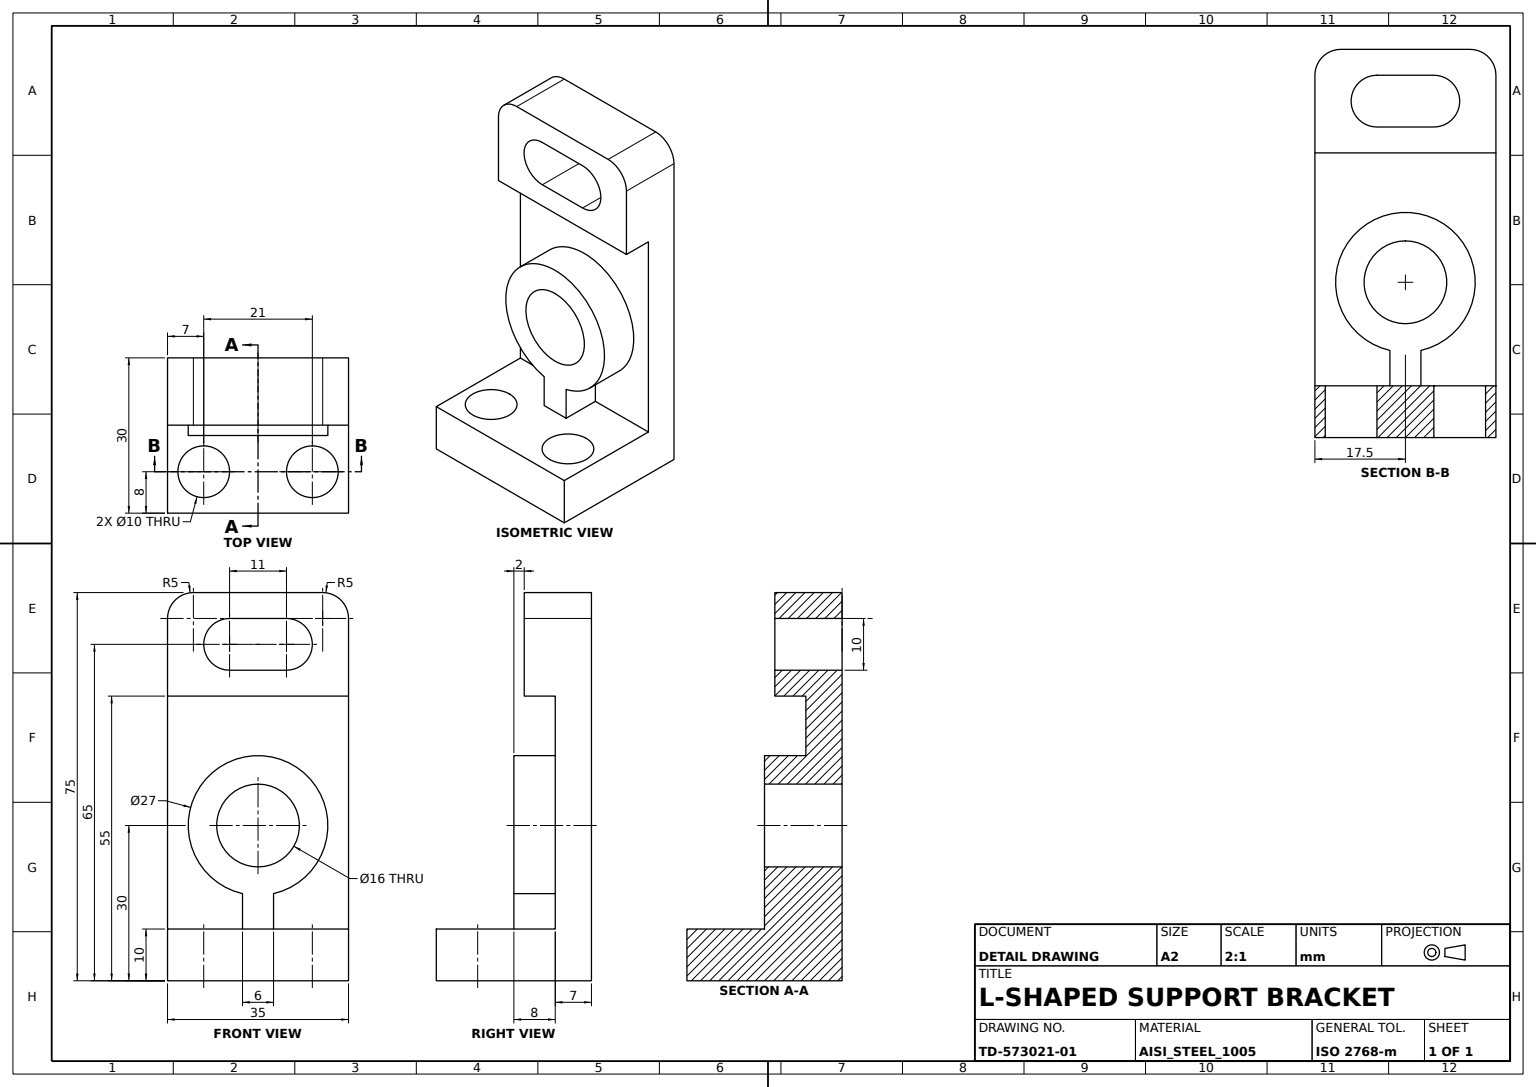
ISO-10303-21;
HEADER;
FILE_DESCRIPTION((''),'2;1');
FILE_NAME('','',(''),(''),'','','');
FILE_SCHEMA(('AUTOMOTIVE_DESIGN'));
ENDSEC;
DATA;
#1=APPLICATION_CONTEXT('');
#2=PRODUCT_CONTEXT('',#1,'mechanical');
#3=PRODUCT('','','',(#2));
#4=PRODUCT_DEFINITION_FORMATION('','',#3);
#5=PRODUCT_DEFINITION_CONTEXT('',#1,'design');
#6=PRODUCT_DEFINITION('','',#4,#5);
#7=PRODUCT_DEFINITION_SHAPE('','',#6);
#8=(LENGTH_UNIT()NAMED_UNIT(*)SI_UNIT(.MILLI.,.METRE.));
#9=(NAMED_UNIT(*)PLANE_ANGLE_UNIT()SI_UNIT($,.RADIAN.));
#10=(NAMED_UNIT(*)SI_UNIT($,.STERADIAN.)SOLID_ANGLE_UNIT());
#11=UNCERTAINTY_MEASURE_WITH_UNIT(LENGTH_MEASURE(0.005),#8,'distance_accuracy_value','');
#12=(GEOMETRIC_REPRESENTATION_CONTEXT(3)GLOBAL_UNCERTAINTY_ASSIGNED_CONTEXT((#11))GLOBAL_UNIT_ASSIGNED_CONTEXT((#8,#9,#10))REPRESENTATION_CONTEXT('',''));
#13=CARTESIAN_POINT('',(-8.,-3.,10.));
#14=VERTEX_POINT('',#13);
#15=CARTESIAN_POINT('',(-8.,-3.,16.837553));
#16=VERTEX_POINT('',#15);
#17=DIRECTION('',(0.,0.,1.));
#18=VECTOR('',#17,1000.);
#19=LINE('',#13,#18);
#20=EDGE_CURVE('',#14,#16,#19,.T.);
#21=ORIENTED_EDGE('',*,*,#20,.F.);
#22=CARTESIAN_POINT('',(0.,-3.,10.));
#23=VERTEX_POINT('',#22);
#24=DIRECTION('',(-1.,0.,0.));
#25=VECTOR('',#24,1000.);
#26=LINE('',#22,#25);
#27=EDGE_CURVE('',#23,#14,#26,.T.);
#28=ORIENTED_EDGE('',*,*,#27,.F.);
#29=CARTESIAN_POINT('',(0.,-3.,16.837553));
#30=VERTEX_POINT('',#29);
#31=LINE('',#22,#18);
#32=EDGE_CURVE('',#23,#30,#31,.T.);
#33=ORIENTED_EDGE('',*,*,#32,.T.);
#34=LINE('',#29,#25);
#35=EDGE_CURVE('',#30,#16,#34,.T.);
#36=ORIENTED_EDGE('',*,*,#35,.T.);
#37=EDGE_LOOP('',(#21,#28,#33,#36));
#38=FACE_BOUND('',#37,.T.);
#39=DIRECTION('',(0.,-1.,0.));
#40=DIRECTION('',(0.,0.,-1.));
#41=AXIS2_PLACEMENT_3D('',#22,#39,#40);
#42=PLANE('',#41);
#43=ADVANCED_FACE('',(#38),#42,.T.);
#44=CARTESIAN_POINT('',(-2.,-5.5,60.));
#45=VERTEX_POINT('',#44);
#46=CARTESIAN_POINT('',(-2.,5.5,60.));
#47=VERTEX_POINT('',#46);
#48=CARTESIAN_POINT('',(-2.,0.,60.));
#49=DIRECTION('',(0.,1.,0.));
#50=VECTOR('',#49,1000.);
#51=LINE('',#48,#50);
#52=EDGE_CURVE('',#45,#47,#51,.T.);
#53=ORIENTED_EDGE('',*,*,#52,.T.);
#54=CARTESIAN_POINT('',(-15.,5.5,60.));
#55=VERTEX_POINT('',#54);
#56=CARTESIAN_POINT('',(9.,5.5,60.));
#57=LINE('',#56,#25);
#58=EDGE_CURVE('',#55,#47,#57,.F.);
#59=ORIENTED_EDGE('',*,*,#58,.F.);
#60=CARTESIAN_POINT('',(-15.,-5.5,60.));
#61=VERTEX_POINT('',#60);
#62=CARTESIAN_POINT('',(-15.,-17.5,60.));
#63=LINE('',#62,#50);
#64=EDGE_CURVE('',#61,#55,#63,.T.);
#65=ORIENTED_EDGE('',*,*,#64,.F.);
#66=CARTESIAN_POINT('',(9.,-5.5,60.));
#67=LINE('',#66,#25);
#68=EDGE_CURVE('',#61,#45,#67,.F.);
#69=ORIENTED_EDGE('',*,*,#68,.T.);
#70=EDGE_LOOP('',(#53,#59,#65,#69));
#71=FACE_BOUND('',#70,.T.);
#72=AXIS2_PLACEMENT_3D('',#56,#40,#24);
#73=PLANE('',#72);
#74=ADVANCED_FACE('',(#71),#73,.F.);
#75=CARTESIAN_POINT('',(2.,10.5,10.));
#76=VERTEX_POINT('',#75);
#77=CARTESIAN_POINT('',(7.,10.5,10.));
#78=AXIS2_PLACEMENT_3D('',#77,#40,#24);
#79=CIRCLE('',#78,5.);
#80=EDGE_CURVE('',#76,#76,#79,.T.);
#81=ORIENTED_EDGE('',*,*,#80,.F.);
#82=EDGE_LOOP('',(#81));
#83=FACE_BOUND('',#82,.T.);
#84=CARTESIAN_POINT('',(12.,10.5,0.));
#85=VERTEX_POINT('',#84);
#86=CARTESIAN_POINT('',(7.,10.5,0.));
#87=DIRECTION('',(1.,0.,0.));
#88=AXIS2_PLACEMENT_3D('',#86,#17,#87);
#89=CIRCLE('',#88,5.);
#90=EDGE_CURVE('',#85,#85,#89,.T.);
#91=ORIENTED_EDGE('',*,*,#90,.F.);
#92=EDGE_LOOP('',(#91));
#93=FACE_BOUND('',#92,.T.);
#94=CYLINDRICAL_SURFACE('',#78,5.);
#95=ADVANCED_FACE('',(#83,#93),#94,.F.);
#96=CARTESIAN_POINT('',(-2.,17.5,55.));
#97=VERTEX_POINT('',#96);
#98=CARTESIAN_POINT('',(-8.,17.5,55.));
#99=VERTEX_POINT('',#98);
#100=LINE('',#96,#25);
#101=EDGE_CURVE('',#97,#99,#100,.T.);
#102=ORIENTED_EDGE('',*,*,#101,.F.);
#103=CARTESIAN_POINT('',(-2.,-17.5,55.));
#104=VERTEX_POINT('',#103);
#105=LINE('',#103,#50);
#106=EDGE_CURVE('',#104,#97,#105,.T.);
#107=ORIENTED_EDGE('',*,*,#106,.F.);
#108=CARTESIAN_POINT('',(-8.,-17.5,55.));
#109=VERTEX_POINT('',#108);
#110=LINE('',#103,#25);
#111=EDGE_CURVE('',#104,#109,#110,.T.);
#112=ORIENTED_EDGE('',*,*,#111,.T.);
#113=LINE('',#108,#50);
#114=EDGE_CURVE('',#109,#99,#113,.T.);
#115=ORIENTED_EDGE('',*,*,#114,.T.);
#116=EDGE_LOOP('',(#102,#107,#112,#115));
#117=FACE_BOUND('',#116,.T.);
#118=AXIS2_PLACEMENT_3D('',#103,#17,#87);
#119=PLANE('',#118);
#120=ADVANCED_FACE('',(#117),#119,.F.);
#121=CARTESIAN_POINT('',(15.,-17.5,0.));
#122=VERTEX_POINT('',#121);
#123=CARTESIAN_POINT('',(15.,17.5,0.));
#124=VERTEX_POINT('',#123);
#125=LINE('',#121,#50);
#126=EDGE_CURVE('',#122,#124,#125,.T.);
#127=ORIENTED_EDGE('',*,*,#126,.T.);
#128=CARTESIAN_POINT('',(15.,17.5,10.));
#129=VERTEX_POINT('',#128);
#130=LINE('',#123,#18);
#131=EDGE_CURVE('',#124,#129,#130,.T.);
#132=ORIENTED_EDGE('',*,*,#131,.T.);
#133=CARTESIAN_POINT('',(15.,-17.5,10.));
#134=VERTEX_POINT('',#133);
#135=LINE('',#133,#50);
#136=EDGE_CURVE('',#134,#129,#135,.T.);
#137=ORIENTED_EDGE('',*,*,#136,.F.);
#138=LINE('',#121,#18);
#139=EDGE_CURVE('',#122,#134,#138,.T.);
#140=ORIENTED_EDGE('',*,*,#139,.F.);
#141=EDGE_LOOP('',(#127,#132,#137,#140));
#142=FACE_BOUND('',#141,.T.);
#143=AXIS2_PLACEMENT_3D('',#121,#24,#17);
#144=PLANE('',#143);
#145=ADVANCED_FACE('',(#142),#144,.F.);
#146=CARTESIAN_POINT('',(-2.,-17.5,70.));
#147=VERTEX_POINT('',#146);
#148=CARTESIAN_POINT('',(-2.,-17.5,75.));
#149=VECTOR('',#40,1000.);
#150=LINE('',#148,#149);
#151=EDGE_CURVE('',#147,#104,#150,.T.);
#152=ORIENTED_EDGE('',*,*,#151,.F.);
#153=CARTESIAN_POINT('',(-15.,-17.5,70.));
#154=VERTEX_POINT('',#153);
#155=LINE('',#153,#25);
#156=EDGE_CURVE('',#147,#154,#155,.T.);
#157=ORIENTED_EDGE('',*,*,#156,.T.);
#158=CARTESIAN_POINT('',(-15.,-17.5,0.));
#159=VERTEX_POINT('',#158);
#160=CARTESIAN_POINT('',(-15.,-17.5,55.));
#161=LINE('',#160,#149);
#162=EDGE_CURVE('',#154,#159,#161,.T.);
#163=ORIENTED_EDGE('',*,*,#162,.T.);
#164=VECTOR('',#87,1000.);
#165=LINE('',#158,#164);
#166=EDGE_CURVE('',#159,#122,#165,.T.);
#167=ORIENTED_EDGE('',*,*,#166,.T.);
#168=ORIENTED_EDGE('',*,*,#139,.T.);
#169=CARTESIAN_POINT('',(-8.,-17.5,10.));
#170=VERTEX_POINT('',#169);
#171=LINE('',#133,#25);
#172=EDGE_CURVE('',#134,#170,#171,.T.);
#173=ORIENTED_EDGE('',*,*,#172,.T.);
#174=LINE('',#169,#18);
#175=EDGE_CURVE('',#170,#109,#174,.T.);
#176=ORIENTED_EDGE('',*,*,#175,.T.);
#177=ORIENTED_EDGE('',*,*,#111,.F.);
#178=EDGE_LOOP('',(#152,#157,#163,#167,#168,#173,#176,#177));
#179=FACE_BOUND('',#178,.T.);
#180=CARTESIAN_POINT('',(0.,-17.5,0.));
#181=AXIS2_PLACEMENT_3D('',#180,#39,#40);
#182=PLANE('',#181);
#183=ADVANCED_FACE('',(#179),#182,.T.);
#184=CARTESIAN_POINT('',(0.,3.,10.));
#185=VERTEX_POINT('',#184);
#186=CARTESIAN_POINT('',(-8.,3.,10.));
#187=VERTEX_POINT('',#186);
#188=LINE('',#184,#25);
#189=EDGE_CURVE('',#185,#187,#188,.T.);
#190=ORIENTED_EDGE('',*,*,#189,.T.);
#191=CARTESIAN_POINT('',(-8.,3.,16.837553));
#192=VERTEX_POINT('',#191);
#193=LINE('',#191,#149);
#194=EDGE_CURVE('',#192,#187,#193,.T.);
#195=ORIENTED_EDGE('',*,*,#194,.F.);
#196=CARTESIAN_POINT('',(0.,3.,16.837553));
#197=VERTEX_POINT('',#196);
#198=LINE('',#196,#25);
#199=EDGE_CURVE('',#197,#192,#198,.T.);
#200=ORIENTED_EDGE('',*,*,#199,.F.);
#201=LINE('',#196,#149);
#202=EDGE_CURVE('',#197,#185,#201,.T.);
#203=ORIENTED_EDGE('',*,*,#202,.T.);
#204=EDGE_LOOP('',(#190,#195,#200,#203));
#205=FACE_BOUND('',#204,.T.);
#206=AXIS2_PLACEMENT_3D('',#196,#49,#17);
#207=PLANE('',#206);
#208=ADVANCED_FACE('',(#205),#207,.T.);
#209=CARTESIAN_POINT('',(0.,0.,30.));
#210=AXIS2_PLACEMENT_3D('',#209,#24,#49);
#211=CIRCLE('',#210,13.5);
#212=EDGE_CURVE('',#30,#197,#211,.T.);
#213=ORIENTED_EDGE('',*,*,#212,.F.);
#214=ORIENTED_EDGE('',*,*,#32,.F.);
#215=VECTOR('',#39,1000.);
#216=LINE('',#184,#215);
#217=EDGE_CURVE('',#185,#23,#216,.T.);
#218=ORIENTED_EDGE('',*,*,#217,.F.);
#219=ORIENTED_EDGE('',*,*,#202,.F.);
#220=EDGE_LOOP('',(#213,#214,#218,#219));
#221=FACE_BOUND('',#220,.T.);
#222=CARTESIAN_POINT('',(0.,0.,38.));
#223=VERTEX_POINT('',#222);
#224=AXIS2_PLACEMENT_3D('',#209,#24,#17);
#225=CIRCLE('',#224,8.);
#226=EDGE_CURVE('',#223,#223,#225,.T.);
#227=ORIENTED_EDGE('',*,*,#226,.T.);
#228=EDGE_LOOP('',(#227));
#229=FACE_BOUND('',#228,.T.);
#230=PLANE('',#224);
#231=ADVANCED_FACE('',(#221,#229),#230,.F.);
#232=LINE('',#169,#50);
#233=EDGE_CURVE('',#170,#14,#232,.T.);
#234=ORIENTED_EDGE('',*,*,#233,.T.);
#235=ORIENTED_EDGE('',*,*,#20,.T.);
#236=CARTESIAN_POINT('',(-8.,0.,30.));
#237=AXIS2_PLACEMENT_3D('',#236,#24,#49);
#238=CIRCLE('',#237,13.5);
#239=EDGE_CURVE('',#16,#192,#238,.T.);
#240=ORIENTED_EDGE('',*,*,#239,.T.);
#241=ORIENTED_EDGE('',*,*,#194,.T.);
#242=CARTESIAN_POINT('',(-8.,17.5,10.));
#243=VERTEX_POINT('',#242);
#244=EDGE_CURVE('',#187,#243,#232,.T.);
#245=ORIENTED_EDGE('',*,*,#244,.T.);
#246=LINE('',#242,#18);
#247=EDGE_CURVE('',#243,#99,#246,.T.);
#248=ORIENTED_EDGE('',*,*,#247,.T.);
#249=ORIENTED_EDGE('',*,*,#114,.F.);
#250=ORIENTED_EDGE('',*,*,#175,.F.);
#251=EDGE_LOOP('',(#234,#235,#240,#241,#245,#248,#249,#250));
#252=FACE_BOUND('',#251,.T.);
#253=AXIS2_PLACEMENT_3D('',#169,#24,#17);
#254=PLANE('',#253);
#255=ADVANCED_FACE('',(#252),#254,.F.);
#256=CARTESIAN_POINT('',(-15.,17.5,70.));
#257=VERTEX_POINT('',#256);
#258=CARTESIAN_POINT('',(-2.,17.5,70.));
#259=VERTEX_POINT('',#258);
#260=CARTESIAN_POINT('',(0.,17.5,70.));
#261=LINE('',#260,#25);
#262=EDGE_CURVE('',#257,#259,#261,.F.);
#263=ORIENTED_EDGE('',*,*,#262,.F.);
#264=CARTESIAN_POINT('',(-15.,12.5,75.));
#265=VERTEX_POINT('',#264);
#266=CARTESIAN_POINT('',(-15.,12.5,70.));
#267=AXIS2_PLACEMENT_3D('',#266,#87,#40);
#268=CIRCLE('',#267,5.);
#269=EDGE_CURVE('',#265,#257,#268,.F.);
#270=ORIENTED_EDGE('',*,*,#269,.F.);
#271=CARTESIAN_POINT('',(-2.,12.5,75.));
#272=VERTEX_POINT('',#271);
#273=LINE('',#271,#25);
#274=EDGE_CURVE('',#272,#265,#273,.T.);
#275=ORIENTED_EDGE('',*,*,#274,.F.);
#276=CARTESIAN_POINT('',(-2.,12.5,70.));
#277=AXIS2_PLACEMENT_3D('',#276,#87,#40);
#278=CIRCLE('',#277,5.);
#279=EDGE_CURVE('',#259,#272,#278,.T.);
#280=ORIENTED_EDGE('',*,*,#279,.F.);
#281=EDGE_LOOP('',(#263,#270,#275,#280));
#282=FACE_BOUND('',#281,.T.);
#283=AXIS2_PLACEMENT_3D('',#276,#24,#17);
#284=CYLINDRICAL_SURFACE('',#283,5.);
#285=ADVANCED_FACE('',(#282),#284,.T.);
#286=CARTESIAN_POINT('',(-2.,-12.5,75.));
#287=VERTEX_POINT('',#286);
#288=CARTESIAN_POINT('',(-2.,17.5,75.));
#289=LINE('',#288,#215);
#290=EDGE_CURVE('',#272,#287,#289,.T.);
#291=ORIENTED_EDGE('',*,*,#290,.F.);
#292=ORIENTED_EDGE('',*,*,#274,.T.);
#293=CARTESIAN_POINT('',(-15.,-12.5,75.));
#294=VERTEX_POINT('',#293);
#295=CARTESIAN_POINT('',(-15.,17.5,75.));
#296=LINE('',#295,#215);
#297=EDGE_CURVE('',#265,#294,#296,.T.);
#298=ORIENTED_EDGE('',*,*,#297,.T.);
#299=LINE('',#286,#25);
#300=EDGE_CURVE('',#294,#287,#299,.F.);
#301=ORIENTED_EDGE('',*,*,#300,.T.);
#302=EDGE_LOOP('',(#291,#292,#298,#301));
#303=FACE_BOUND('',#302,.T.);
#304=AXIS2_PLACEMENT_3D('',#288,#40,#24);
#305=PLANE('',#304);
#306=ADVANCED_FACE('',(#303),#305,.F.);
#307=CARTESIAN_POINT('',(-15.,17.5,0.));
#308=VERTEX_POINT('',#307);
#309=LINE('',#307,#164);
#310=EDGE_CURVE('',#308,#124,#309,.T.);
#311=ORIENTED_EDGE('',*,*,#310,.T.);
#312=ORIENTED_EDGE('',*,*,#126,.F.);
#313=ORIENTED_EDGE('',*,*,#166,.F.);
#314=LINE('',#158,#50);
#315=EDGE_CURVE('',#159,#308,#314,.T.);
#316=ORIENTED_EDGE('',*,*,#315,.T.);
#317=EDGE_LOOP('',(#311,#312,#313,#316));
#318=FACE_BOUND('',#317,.T.);
#319=CARTESIAN_POINT('',(12.,-10.5,0.));
#320=VERTEX_POINT('',#319);
#321=CARTESIAN_POINT('',(7.,-10.5,0.));
#322=AXIS2_PLACEMENT_3D('',#321,#17,#87);
#323=CIRCLE('',#322,5.);
#324=EDGE_CURVE('',#320,#320,#323,.T.);
#325=ORIENTED_EDGE('',*,*,#324,.T.);
#326=EDGE_LOOP('',(#325));
#327=FACE_BOUND('',#326,.T.);
#328=ORIENTED_EDGE('',*,*,#90,.T.);
#329=EDGE_LOOP('',(#328));
#330=FACE_BOUND('',#329,.T.);
#331=AXIS2_PLACEMENT_3D('',#158,#17,#87);
#332=PLANE('',#331);
#333=ADVANCED_FACE('',(#318,#327,#330),#332,.F.);
#334=LINE('',#128,#25);
#335=EDGE_CURVE('',#129,#243,#334,.T.);
#336=ORIENTED_EDGE('',*,*,#335,.F.);
#337=ORIENTED_EDGE('',*,*,#131,.F.);
#338=ORIENTED_EDGE('',*,*,#310,.F.);
#339=CARTESIAN_POINT('',(-15.,17.5,55.));
#340=LINE('',#339,#149);
#341=EDGE_CURVE('',#257,#308,#340,.T.);
#342=ORIENTED_EDGE('',*,*,#341,.F.);
#343=ORIENTED_EDGE('',*,*,#262,.T.);
#344=LINE('',#96,#18);
#345=EDGE_CURVE('',#97,#259,#344,.T.);
#346=ORIENTED_EDGE('',*,*,#345,.F.);
#347=ORIENTED_EDGE('',*,*,#101,.T.);
#348=ORIENTED_EDGE('',*,*,#247,.F.);
#349=EDGE_LOOP('',(#336,#337,#338,#342,#343,#346,#347,#348));
#350=FACE_BOUND('',#349,.T.);
#351=CARTESIAN_POINT('',(0.,17.5,0.));
#352=AXIS2_PLACEMENT_3D('',#351,#39,#40);
#353=PLANE('',#352);
#354=ADVANCED_FACE('',(#350),#353,.F.);
#355=CARTESIAN_POINT('',(-15.,0.,22.));
#356=VERTEX_POINT('',#355);
#357=CARTESIAN_POINT('',(-15.,0.,30.));
#358=AXIS2_PLACEMENT_3D('',#357,#87,#40);
#359=CIRCLE('',#358,8.);
#360=EDGE_CURVE('',#356,#356,#359,.T.);
#361=ORIENTED_EDGE('',*,*,#360,.F.);
#362=EDGE_LOOP('',(#361));
#363=FACE_BOUND('',#362,.T.);
#364=ORIENTED_EDGE('',*,*,#226,.F.);
#365=EDGE_LOOP('',(#364));
#366=FACE_BOUND('',#365,.T.);
#367=CYLINDRICAL_SURFACE('',#224,8.);
#368=ADVANCED_FACE('',(#363,#366),#367,.F.);
#369=ORIENTED_EDGE('',*,*,#80,.T.);
#370=EDGE_LOOP('',(#369));
#371=FACE_BOUND('',#370,.T.);
#372=ORIENTED_EDGE('',*,*,#136,.T.);
#373=ORIENTED_EDGE('',*,*,#335,.T.);
#374=ORIENTED_EDGE('',*,*,#244,.F.);
#375=ORIENTED_EDGE('',*,*,#189,.F.);
#376=ORIENTED_EDGE('',*,*,#217,.T.);
#377=ORIENTED_EDGE('',*,*,#27,.T.);
#378=ORIENTED_EDGE('',*,*,#233,.F.);
#379=ORIENTED_EDGE('',*,*,#172,.F.);
#380=EDGE_LOOP('',(#372,#373,#374,#375,#376,#377,#378,#379));
#381=FACE_BOUND('',#380,.T.);
#382=CARTESIAN_POINT('',(2.,-10.5,10.));
#383=VERTEX_POINT('',#382);
#384=CARTESIAN_POINT('',(7.,-10.5,10.));
#385=AXIS2_PLACEMENT_3D('',#384,#40,#24);
#386=CIRCLE('',#385,5.);
#387=EDGE_CURVE('',#383,#383,#386,.T.);
#388=ORIENTED_EDGE('',*,*,#387,.T.);
#389=EDGE_LOOP('',(#388));
#390=FACE_BOUND('',#389,.T.);
#391=AXIS2_PLACEMENT_3D('',#133,#40,#24);
#392=PLANE('',#391);
#393=ADVANCED_FACE('',(#371,#381,#390),#392,.F.);
#394=ORIENTED_EDGE('',*,*,#239,.F.);
#395=ORIENTED_EDGE('',*,*,#35,.F.);
#396=ORIENTED_EDGE('',*,*,#212,.T.);
#397=ORIENTED_EDGE('',*,*,#199,.T.);
#398=EDGE_LOOP('',(#394,#395,#396,#397));
#399=FACE_BOUND('',#398,.T.);
#400=CYLINDRICAL_SURFACE('',#224,13.5);
#401=ADVANCED_FACE('',(#399),#400,.T.);
#402=ORIENTED_EDGE('',*,*,#324,.F.);
#403=EDGE_LOOP('',(#402));
#404=FACE_BOUND('',#403,.T.);
#405=ORIENTED_EDGE('',*,*,#387,.F.);
#406=EDGE_LOOP('',(#405));
#407=FACE_BOUND('',#406,.T.);
#408=CYLINDRICAL_SURFACE('',#385,5.);
#409=ADVANCED_FACE('',(#404,#407),#408,.F.);
#410=CARTESIAN_POINT('',(-2.,-5.5,70.));
#411=VERTEX_POINT('',#410);
#412=CARTESIAN_POINT('',(-2.,-5.5,65.));
#413=AXIS2_PLACEMENT_3D('',#412,#87,#40);
#414=CIRCLE('',#413,5.);
#415=EDGE_CURVE('',#411,#45,#414,.T.);
#416=ORIENTED_EDGE('',*,*,#415,.F.);
#417=CARTESIAN_POINT('',(-2.,5.5,70.));
#418=VERTEX_POINT('',#417);
#419=CARTESIAN_POINT('',(-2.,0.,70.));
#420=LINE('',#419,#215);
#421=EDGE_CURVE('',#418,#411,#420,.T.);
#422=ORIENTED_EDGE('',*,*,#421,.F.);
#423=CARTESIAN_POINT('',(-2.,5.5,65.));
#424=AXIS2_PLACEMENT_3D('',#423,#87,#40);
#425=CIRCLE('',#424,5.);
#426=EDGE_CURVE('',#47,#418,#425,.T.);
#427=ORIENTED_EDGE('',*,*,#426,.F.);
#428=ORIENTED_EDGE('',*,*,#52,.F.);
#429=EDGE_LOOP('',(#416,#422,#427,#428));
#430=FACE_BOUND('',#429,.T.);
#431=ORIENTED_EDGE('',*,*,#290,.T.);
#432=CARTESIAN_POINT('',(-2.,-12.5,70.));
#433=AXIS2_PLACEMENT_3D('',#432,#87,#40);
#434=CIRCLE('',#433,5.);
#435=EDGE_CURVE('',#287,#147,#434,.T.);
#436=ORIENTED_EDGE('',*,*,#435,.T.);
#437=ORIENTED_EDGE('',*,*,#151,.T.);
#438=ORIENTED_EDGE('',*,*,#106,.T.);
#439=ORIENTED_EDGE('',*,*,#345,.T.);
#440=ORIENTED_EDGE('',*,*,#279,.T.);
#441=EDGE_LOOP('',(#431,#436,#437,#438,#439,#440));
#442=FACE_BOUND('',#441,.T.);
#443=CARTESIAN_POINT('',(-2.,0.,0.));
#444=AXIS2_PLACEMENT_3D('',#443,#87,#40);
#445=PLANE('',#444);
#446=ADVANCED_FACE('',(#430,#442),#445,.T.);
#447=ORIENTED_EDGE('',*,*,#297,.F.);
#448=ORIENTED_EDGE('',*,*,#269,.T.);
#449=ORIENTED_EDGE('',*,*,#341,.T.);
#450=ORIENTED_EDGE('',*,*,#315,.F.);
#451=ORIENTED_EDGE('',*,*,#162,.F.);
#452=CARTESIAN_POINT('',(-15.,-12.5,70.));
#453=AXIS2_PLACEMENT_3D('',#452,#87,#40);
#454=CIRCLE('',#453,5.);
#455=EDGE_CURVE('',#154,#294,#454,.F.);
#456=ORIENTED_EDGE('',*,*,#455,.T.);
#457=EDGE_LOOP('',(#447,#448,#449,#450,#451,#456));
#458=FACE_BOUND('',#457,.T.);
#459=CARTESIAN_POINT('',(-15.,5.5,70.));
#460=VERTEX_POINT('',#459);
#461=CARTESIAN_POINT('',(-15.,5.5,65.));
#462=AXIS2_PLACEMENT_3D('',#461,#87,#40);
#463=CIRCLE('',#462,5.);
#464=EDGE_CURVE('',#55,#460,#463,.T.);
#465=ORIENTED_EDGE('',*,*,#464,.T.);
#466=CARTESIAN_POINT('',(-15.,-5.5,70.));
#467=VERTEX_POINT('',#466);
#468=LINE('',#153,#215);
#469=EDGE_CURVE('',#460,#467,#468,.T.);
#470=ORIENTED_EDGE('',*,*,#469,.T.);
#471=CARTESIAN_POINT('',(-15.,-5.5,65.));
#472=AXIS2_PLACEMENT_3D('',#471,#87,#40);
#473=CIRCLE('',#472,5.);
#474=EDGE_CURVE('',#467,#61,#473,.T.);
#475=ORIENTED_EDGE('',*,*,#474,.T.);
#476=ORIENTED_EDGE('',*,*,#64,.T.);
#477=EDGE_LOOP('',(#465,#470,#475,#476));
#478=FACE_BOUND('',#477,.T.);
#479=ORIENTED_EDGE('',*,*,#360,.T.);
#480=EDGE_LOOP('',(#479));
#481=FACE_BOUND('',#480,.T.);
#482=AXIS2_PLACEMENT_3D('',#160,#87,#40);
#483=PLANE('',#482);
#484=ADVANCED_FACE('',(#458,#478,#481),#483,.F.);
#485=ORIENTED_EDGE('',*,*,#464,.F.);
#486=ORIENTED_EDGE('',*,*,#58,.T.);
#487=ORIENTED_EDGE('',*,*,#426,.T.);
#488=CARTESIAN_POINT('',(9.,5.5,70.));
#489=LINE('',#488,#25);
#490=EDGE_CURVE('',#460,#418,#489,.F.);
#491=ORIENTED_EDGE('',*,*,#490,.F.);
#492=EDGE_LOOP('',(#485,#486,#487,#491));
#493=FACE_BOUND('',#492,.T.);
#494=CARTESIAN_POINT('',(9.,5.5,65.));
#495=AXIS2_PLACEMENT_3D('',#494,#24,#17);
#496=CYLINDRICAL_SURFACE('',#495,5.);
#497=ADVANCED_FACE('',(#493),#496,.F.);
#498=ORIENTED_EDGE('',*,*,#490,.T.);
#499=ORIENTED_EDGE('',*,*,#421,.T.);
#500=CARTESIAN_POINT('',(9.,-5.5,70.));
#501=LINE('',#500,#25);
#502=EDGE_CURVE('',#467,#411,#501,.F.);
#503=ORIENTED_EDGE('',*,*,#502,.F.);
#504=ORIENTED_EDGE('',*,*,#469,.F.);
#505=EDGE_LOOP('',(#498,#499,#503,#504));
#506=FACE_BOUND('',#505,.T.);
#507=AXIS2_PLACEMENT_3D('',#500,#17,#87);
#508=PLANE('',#507);
#509=ADVANCED_FACE('',(#506),#508,.F.);
#510=ORIENTED_EDGE('',*,*,#502,.T.);
#511=ORIENTED_EDGE('',*,*,#415,.T.);
#512=ORIENTED_EDGE('',*,*,#68,.F.);
#513=ORIENTED_EDGE('',*,*,#474,.F.);
#514=EDGE_LOOP('',(#510,#511,#512,#513));
#515=FACE_BOUND('',#514,.T.);
#516=CARTESIAN_POINT('',(9.,-5.5,65.));
#517=AXIS2_PLACEMENT_3D('',#516,#24,#17);
#518=CYLINDRICAL_SURFACE('',#517,5.);
#519=ADVANCED_FACE('',(#515),#518,.F.);
#520=ORIENTED_EDGE('',*,*,#455,.F.);
#521=ORIENTED_EDGE('',*,*,#156,.F.);
#522=ORIENTED_EDGE('',*,*,#435,.F.);
#523=ORIENTED_EDGE('',*,*,#300,.F.);
#524=EDGE_LOOP('',(#520,#521,#522,#523));
#525=FACE_BOUND('',#524,.T.);
#526=CARTESIAN_POINT('',(0.,-12.5,70.));
#527=AXIS2_PLACEMENT_3D('',#526,#87,#40);
#528=CYLINDRICAL_SURFACE('',#527,5.);
#529=ADVANCED_FACE('',(#525),#528,.T.);
#530=CLOSED_SHELL('',(#43,#74,#95,#120,#145,#183,#208,#231,#255,#285,#306,#333,#354,#368,#393,#401,#409,#446,#484,#497,#509,#519,#529));
#531=MANIFOLD_SOLID_BREP('',#530);
#532=ADVANCED_BREP_SHAPE_REPRESENTATION('',(#531),#12);
#533=SHAPE_DEFINITION_REPRESENTATION(#7,#532);
ENDSEC;
END-ISO-10303-21;
